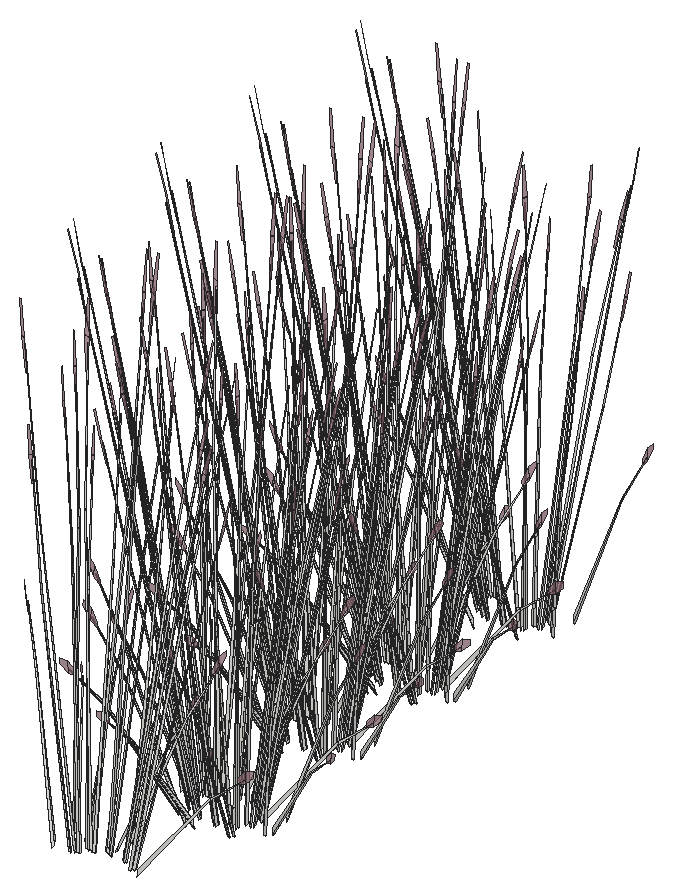
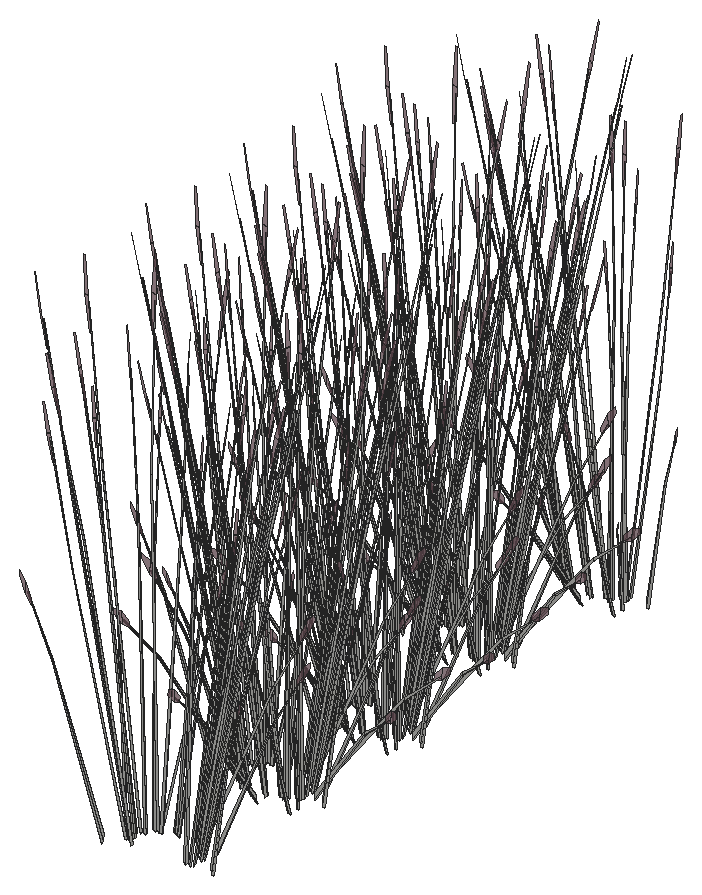
# SketchUp Ruby script. Lengths in inches.
U = 1.inch
M = Sketchup.active_model
def pt(a) = Geom::Point3d.new(a.map { |v| v * U })
def face(e, loops, mat)
  f = e.add_face(loops[0].map { |a| pt(a) })
  loops[1..].each { |l| e.add_face(l.map { |a| pt(a) }).erase! }
  f.material = f.back_material = mat if mat
  f
end
# faces: each face lists its corners as indices into pts; further lists are holes
def faces(e, pts, list, mat = nil) = list.each { |f| face(e, (f[0].is_a?(Array) ? f : [f]).map { |l| l.map { |i| pts[i] } }, mat) }
# xy, xz, yz: faces in a plane at the given z, y or x. An outline is a flat list of corners, or four numbers for a rectangle; further outlines are holes
def ring(l) = l.size == 4 ? [[l[0], l[1]], [l[2], l[1]], [l[2], l[3]], [l[0], l[3]]] : l.each_slice(2).to_a
def flat(e, list, mat, &to3) = list.each { |f| face(e, (f[0].is_a?(Array) ? f : [f]).map { |l| ring(l).map { |u, v| to3.(u, v) } }, mat) }
def xy(e, z, list, mat = nil) = flat(e, list, mat) { |x, y| [x, y, z] }
def xz(e, y, list, mat = nil) = flat(e, list, mat) { |x, z| [x, y, z] }
def yz(e, x, list, mat = nil) = flat(e, list, mat) { |y, z| [x, y, z] }
def lines(e, pts, list) = list.each { |a, b| e.add_line(pt(pts[a]), pt(pts[b])) }
# prism: a flat outline (further loops are holes) pulled along v
def prism(e, loops, v, mat = nil)
  f = face(e, loops, mat); d = Geom::Vector3d.new(v.map { |x| x * U })
  f.pushpull(f.normal.samedirection?(d) ? d.length : -d.length)
end
def box(e, o, s, mat = nil) = prism(e, [[o, [o[0] + s[0], o[1], o[2]], [o[0] + s[0], o[1] + s[1], o[2]], [o[0], o[1] + s[1], o[2]]]], [0, 0, s[2]], mat)
def at(x, y, z, deg = 0) = Geom::Transformation.translation(pt([x, y, z])) * Geom::Transformation.rotation(ORIGIN, Z_AXIS, deg.degrees)
def axes(o, x, y, z) = Geom::Transformation.new([*x, 0, *y, 0, *z, 0, *pt(o).to_a, 1])
def part(name) = M.definitions.add(name)
# library, detail: a bought-in or finely detailed component or shape, given as its bounding box
def library(name, o, s) = part(name).tap { |d| box(d.entities, o, s) }
def detail(e, o, s) = box(e.add_group.entities, o, s)
def put(e, d, t, mat = nil) = e.add_instance(d, t).tap { |i| i.material = mat if mat }
def group(e, t, mat = nil) = e.add_group.tap { |g| g.transformation = t; g.material = mat if mat }.entities
root = M.entities
M.materials.add("LightPink_Translucent").color = [144, 107, 117]
M.materials["LightPink_Translucent"].alpha = 0.75
c1 = part("blade")
p = [[2.15,0.21,22],[0,0.17,0],[0.09,0.45,0],[2.18,0.31,22],[2.29,0.31,22],[0.38,0.45,0],
  [2.48,0.24,33],[2.49,0.24,33],[2.48,0.22,33]]
faces(c1.entities,p,[[0,1,2,3],[4,5,2,3],[6,3,4,7],[8,0,3,6]])
c2 = part("seeds")
p = [[0.3,-0.1,1.38],[-0.01,-0.03,1.59],[-0.01,-0.03,0.03],[0.14,-0.07,-0.07],[0.29,-0.03,3],[0.15,0.01,3.11]]
faces(c2.entities,p,[[0,1,2,3],[1,0,4,5]],"LightPink_Translucent")
c3 = part("blade with seeds")
put(c3.entities,c1,at(0,0,0))
put(c3.entities,c2,axes([2.4,0.25,30.99],[1.5799,-0.05474,1.17369],[-0.12525,1.92788,0.29478],[-0.07173,-0.02425,1.56792]))
put(root,c3,axes([335.36,424.53,52.46],[-0.28729,-0.24465,0.31292],[0.32804,-0.23159,-0.40398],[0.16667,0.03524,0.77298]))
put(root,c3,axes([335.88,424.44,52.17],[0.10831,-0.00661,1.54581],[0.29709,-0.30358,-0.24447],[0.19266,0.04007,0.12397]))
put(root,c3,axes([331.55,424.15,52.18],[-0.12522,-0.35963,0.42415],[0.49122,-0.06241,0.34973],[-0.14477,0.08458,0.87768]))
put(root,c3,axes([331.45,424.08,52.18],[-0.34663,-0.16434,0.05682],[0.20181,-0.23402,0.44729],[-0.11113,0.07566,0.68204]))
put(root,c3,axes([331.85,424.03,52.46],[0.43951,-0.05584,0.31292],[0.11606,0.31924,-0.40398],[-0.12595,0.08575,0.77298]))
put(root,c3,axes([330.16,423.88,52.16],[0.06444,0.01048,1.56736],[0.19934,0.34525,-0.1481],[-0.13191,0.09062,0.27737]))
put(root,c3,axes([335.62,424.75,52.18],[-0.02542,0.29714,0.05682],[-0.38391,-0.00815,0.44729],[0.14706,0.03109,0.68204]))
put(root,c3,axes([335.65,424.65,52.18],[-0.3723,0.25748,0.42415],[-0.32109,-0.27343,0.34973],[0.17467,0.04749,0.87768]))
put(root,c3,axes([330.85,424.93,52.99],[0.44556,0.1043,-0.05733],[-0.13706,0.32103,-0.25992],[-0.07288,0.04874,0.85731]))
put(root,c3,axes([334.47,424.95,52.46],[-0.07798,-0.31474,0.31292],[0.44579,-0.08311,-0.40398],[0.11974,0.09019,0.77298]))
put(root,c3,axes([332.45,424.66,52.46],[0.34164,-0.20573,0.31292],[0.3234,0.23491,-0.40398],[-0.04921,0.11936,0.77298]))
put(root,c3,axes([334.04,425.39,52.16],[0.00149,-0.04731,1.56736],[0.4327,-0.20872,-0.1481],[0.1503,0.0745,0.27737]))
put(root,c3,axes([332.14,424.85,52.18],[-0.41493,-0.01821,0.05682],[0.01138,-0.27493,0.44729],[-0.04342,0.10531,0.68204]))
put(root,c3,axes([332.27,424.875,52.18],[-0.35954,-0.26661,0.42415],[0.38183,-0.22994,0.34973],[-0.06632,0.12508,0.87768]))
put(root,c3,axes([333.4,425,52.46],[0.15222,-0.30049,0.31292],[0.44409,0.08764,-0.40398],[0.04072,0.12098,0.77298]))
put(root,c3,axes([334.54,425.24,52.18],[-0.22948,0.24822,0.05682],[-0.32679,-0.14452,0.44729],[0.10565,0.07958,0.68204]))
put(root,c3,axes([334,426.07,52.99],[0.34892,-0.22417,-0.05733],[0.3197,0.24551,-0.25992],[0.02251,0.06957,0.85731]))
put(root,c3,axes([334.64,425.17,52.18],[-0.5022,0.08967,0.42415],[-0.08716,-0.35177,0.34973],[0.11811,0.10367,0.87768]))
put(root,c3,axes([333.27,425.27,52.18],[-0.37205,0.1328,0.05682],[-0.18211,-0.24217,0.44729],[0.03593,0.10675,0.68204]))
put(root,c3,axes([331.09,424.89,52.17],[-0.01255,0.07733,1.54581],[0.35618,0.269,-0.24447],[-0.09325,0.12721,0.12397]))
put(root,c3,axes([332.23,424.72,52.77],[0.55492,0.01936,-0.11927],[-0.01517,0.36657,-0.66198],[-0.03855,0.14118,1.00587]))
put(root,c3,axes([333.4,425.25,52.47],[-0.49753,-0.10215,0.47081],[0.17013,-0.33585,0.3882],[0.0299,0.13207,0.97422]))
put(root,c3,axes([331.05,425.6875,52.16],[0.05728,-0.02359,1.56736],[0.47345,0.15692,-0.1481],[-0.01113,0.13066,0.27737]))
put(root,c3,axes([335.16,430.65,52.17],[-0.07723,-0.05479,1.54581],[-0.51538,0.03473,-0.24447],[-0.08225,-0.13104,0.12397]))
put(root,c3,axes([333.14,425.85,52.17],[0.064,0.06292,1.54581],[0.51651,0.02472,-0.24447],[0.05194,0.13877,0.12397]))
put(root,c3,axes([337.48,431.32,52.17],[-0.00487,-0.07777,1.54581],[-0.41166,-0.22476,-0.24447],[0.06364,-0.13625,0.12397]))
put(root,c3,axes([337.37,431.04,52.16],[-0.05128,0.02985,1.56736],[-0.5024,-0.1007,-0.1481],[-0.01819,-0.13025,0.27737]))
put(root,c3,axes([334.63,430.47,52.16],[-0.00942,0.04684,1.56736],[-0.46458,0.16998,-0.1481],[-0.13671,-0.08689,0.27737]))
put(root,c3,axes([334.53,431.3,52.5],[0.56246,-0.10044,0.47505],[0.09762,0.39398,0.3917],[-0.13228,-0.11611,0.983]))
put(root,c3,axes([335.8,431.375,52.18],[0.49753,0.10215,0.42415],[-0.17013,0.33585,0.34973],[-0.0299,-0.13207,0.87768]))
put(root,c3,axes([335.93,431.35,52.18],[0.37205,-0.1328,0.05682],[0.18211,0.24217,0.44729],[-0.03593,-0.10675,0.68204]))
put(root,c3,axes([334.66,431.39,52.18],[0.22948,-0.24822,0.05682],[0.32679,0.14452,0.44729],[-0.10565,-0.07958,0.68204]))
put(root,c3,axes([335.8,431.62,52.46],[-0.15222,0.30049,0.31292],[-0.44409,-0.08764,-0.40398],[-0.04072,-0.12098,0.77298]))
put(root,c3,axes([336.93,431.75,52.18],[0.35954,0.26661,0.42415],[-0.38183,0.22994,0.34973],[0.06632,-0.12508,0.87768]))
put(root,c3,axes([334.76,431.36,52.8],[-0.33698,0.3746,-0.12034],[-0.48801,-0.21581,-0.66795],[-0.16964,-0.10584,1.01494]))
put(root,c3,axes([337.0625,431.77,52.18],[0.41493,0.01821,0.05682],[-0.01138,0.27493,0.44729],[0.04342,-0.10531,0.68204]))
put(root,c3,axes([336.75,431.96,52.46],[-0.34164,0.20573,0.31292],[-0.3234,-0.23491,-0.40398],[0.04921,-0.11936,0.77298]))
put(root,c3,axes([333.47,431.25,52.17],[-0.10864,-0.00276,1.54581],[-0.34587,0.27582,-0.24447],[-0.18454,-0.05636,0.12397]))
put(root,c3,axes([334.73,431.67,52.46],[0.07798,0.31474,0.31292],[-0.44579,0.08311,-0.40398],[-0.11974,-0.09019,0.77298]))
put(root,c3,axes([333.39,431.875,52.5],[0.41698,-0.28837,0.47505],[0.35962,0.30624,0.3917],[-0.19563,-0.05319,0.983]))
put(root,c3,axes([338.73,432.53,52.16],[-0.06595,-0.00297,1.56736],[-0.27386,-0.31799,-0.1481],[0.10998,-0.10455,0.27737]))
put(root,c3,axes([333.58,431.875,52.18],[0.02542,-0.29714,0.05682],[0.38391,0.00815,0.44729],[-0.14706,-0.03109,0.68204]))
put(root,c3,axes([337.35,432.6,52.46],[-0.43951,0.05584,0.31292],[-0.11606,-0.31924,-0.40398],[0.12595,-0.08575,0.77298]))
put(root,c3,axes([337.75,432.54,52.18],[0.34663,0.16434,0.05682],[-0.20181,0.23402,0.44729],[0.11113,-0.07566,0.68204]))
put(root,c3,axes([337.65,432.48,52.18],[0.12522,0.35963,0.42415],[-0.49122,0.06241,0.34973],[0.14477,-0.08458,0.87768]))
put(root,c3,axes([338.97,432.91,52.17],[0.07006,-0.05952,1.54581],[-0.08968,-0.3651,-0.24447],[0.1758,-0.06922,0.12397]))
put(root,c3,axes([333.05,431.49,52.16],[0.03743,0.039,1.56736],[-0.18045,0.35054,-0.1481],[-0.18276,0.00254,0.27737]))
put(root,c3,axes([333.84,432.1,52.46],[0.28729,0.24465,0.31292],[-0.32804,0.23159,-0.40398],[-0.16667,-0.03524,0.77298]))
put(root,c3,axes([337.42,433.36,52.46],[-0.41962,-0.10901,0.31292],[0.12239,-0.31802,-0.40398],[0.16894,-0.02916,0.77298]))
put(root,c3,axes([333.02,432.78,52.18],[0.14265,-0.35629,0.42415],[0.46898,0.12183,0.34973],[-0.18443,0.02141,0.87768]))
put(root,c3,axes([332.99,432.68,52.18],[-0.18545,-0.26643,0.05682],[0.33817,-0.13041,0.44729],[-0.14907,0.02573,0.68204]))
put(root,c3,axes([337.8,433.46,52.18],[0.18545,0.26643,0.05682],[-0.33817,0.13041,0.44729],[0.14907,-0.02573,0.68204]))
put(root,c3,axes([337.76,433.36,52.18],[-0.14265,0.35629,0.42415],[-0.46898,-0.12183,0.34973],[0.18443,-0.02141,0.87768]))
put(root,c3,axes([333.37,432.78,52.46],[0.41962,0.10901,0.31292],[-0.12239,0.31802,-0.40398],[-0.16894,0.02916,0.77298]))
put(root,c3,axes([338.6,434.52,52.16],[-0.04566,-0.03421,1.56736],[0.09987,-0.36669,-0.1481],[0.17984,-0.02343,0.27737]))
put(root,c3,axes([332.66,433.03,52.17],[-0.08245,0.05073,1.54581],[0.00701,0.37067,-0.24447],[-0.18899,0.0482,0.12397]))
put(root,c3,axes([336.95,434.04,52.46],[-0.28729,-0.24465,0.31292],[0.32804,-0.23159,-0.40398],[0.16667,0.03524,0.77298]))
put(root,c3,axes([337.47,433.96,52.17],[0.10831,-0.00661,1.54581],[0.29709,-0.30358,-0.24447],[0.19266,0.04007,0.12397]))
put(root,c3,axes([333.14,433.66,52.18],[-0.12522,-0.35963,0.42415],[0.49122,-0.06241,0.34973],[-0.14477,0.08458,0.87768]))
put(root,c3,axes([333.04,433.6,52.18],[-0.34663,-0.16434,0.05682],[0.20181,-0.23402,0.44729],[-0.11113,0.07566,0.68204]))
put(root,c3,axes([333.4375,433.55,52.46],[0.43951,-0.05584,0.31292],[0.11606,0.31924,-0.40398],[-0.12595,0.08575,0.77298]))
put(root,c3,axes([331.75,433.4,52.16],[0.06444,0.01048,1.56736],[0.19934,0.34525,-0.1481],[-0.13191,0.09062,0.27737]))
put(root,c3,axes([337.21,434.27,52.18],[-0.02542,0.29714,0.05682],[-0.38391,-0.00815,0.44729],[0.14706,0.03109,0.68204]))
put(root,c3,axes([337.24,434.17,52.18],[-0.3723,0.25748,0.42415],[-0.32109,-0.27343,0.34973],[0.17467,0.04749,0.87768]))
put(root,c3,axes([332.44,434.45,52.99],[0.44556,0.1043,-0.05733],[-0.13706,0.32103,-0.25992],[-0.07288,0.04874,0.85731]))
put(root,c3,axes([336.06,434.47,52.46],[-0.07798,-0.31474,0.31292],[0.44579,-0.08311,-0.40398],[0.11974,0.09019,0.77298]))
put(root,c3,axes([334.03,434.18,52.46],[0.34164,-0.20573,0.31292],[0.3234,0.23491,-0.40398],[-0.04921,0.11936,0.77298]))
put(root,c3,axes([335.62,434.91,52.16],[0.00149,-0.04731,1.56736],[0.4327,-0.20872,-0.1481],[0.1503,0.0745,0.27737]))
put(root,c3,axes([333.72,434.37,52.18],[-0.41493,-0.01821,0.05682],[0.01138,-0.27493,0.44729],[-0.04342,0.10531,0.68204]))
put(root,c3,axes([333.86,434.39,52.18],[-0.35954,-0.26661,0.42415],[0.38183,-0.22994,0.34973],[-0.06632,0.12508,0.87768]))
put(root,c3,axes([334.99,434.52,52.46],[0.15222,-0.30049,0.31292],[0.44409,0.08764,-0.40398],[0.04072,0.12098,0.77298]))
put(root,c3,axes([336.13,434.75,52.18],[-0.22948,0.24822,0.05682],[-0.32679,-0.14452,0.44729],[0.10565,0.07958,0.68204]))
put(root,c3,axes([335.59,435.59,52.99],[0.34892,-0.22417,-0.05733],[0.3197,0.24551,-0.25992],[0.02251,0.06957,0.85731]))
put(root,c3,axes([336.22,434.6875,52.18],[-0.5022,0.08967,0.42415],[-0.08716,-0.35177,0.34973],[0.11811,0.10367,0.87768]))
put(root,c3,axes([334.85,434.79,52.18],[-0.37205,0.1328,0.05682],[-0.18211,-0.24217,0.44729],[0.03593,0.10675,0.68204]))
put(root,c3,axes([332.68,434.41,52.17],[-0.01255,0.07733,1.54581],[0.35618,0.269,-0.24447],[-0.09325,0.12721,0.12397]))
put(root,c3,axes([333.82,434.24,52.77],[0.55492,0.01936,-0.11927],[-0.01517,0.36657,-0.66198],[-0.03855,0.14118,1.00587]))
put(root,c3,axes([334.98,434.77,52.47],[-0.49753,-0.10215,0.47081],[0.17013,-0.33585,0.3882],[0.0299,0.13207,0.97422]))
put(root,c3,axes([332.64,435.2,52.16],[0.05728,-0.02359,1.56736],[0.47345,0.15692,-0.1481],[-0.01113,0.13066,0.27737]))
put(root,c3,axes([334.73,435.37,52.17],[0.064,0.06292,1.54581],[0.51651,0.02472,-0.24447],[0.05194,0.13877,0.12397]))
put(root,c3,axes([333.57,440.52,52.17],[-0.07723,-0.05479,1.54581],[-0.51538,0.03473,-0.24447],[-0.08225,-0.13104,0.12397]))
put(root,c3,axes([335.89,441.1875,52.17],[-0.00487,-0.07777,1.54581],[-0.41166,-0.22476,-0.24447],[0.06364,-0.13625,0.12397]))
put(root,c3,axes([335.78,440.91,52.16],[-0.05128,0.02985,1.56736],[-0.5024,-0.1007,-0.1481],[-0.01819,-0.13025,0.27737]))
put(root,c3,axes([333.05,440.34,52.16],[-0.00942,0.04684,1.56736],[-0.46458,0.16998,-0.1481],[-0.13671,-0.08689,0.27737]))
put(root,c3,axes([332.94,441.17,52.5],[0.56246,-0.10044,0.47505],[0.09762,0.39398,0.3917],[-0.13228,-0.11611,0.983]))
put(root,c3,axes([334.22,441.24,52.18],[0.49753,0.10215,0.42415],[-0.17013,0.33585,0.34973],[-0.0299,-0.13207,0.87768]))
put(root,c3,axes([334.35,441.22,52.18],[0.37205,-0.1328,0.05682],[0.18211,0.24217,0.44729],[-0.03593,-0.10675,0.68204]))
put(root,c3,axes([333.07,441.25,52.18],[0.22948,-0.24822,0.05682],[0.32679,0.14452,0.44729],[-0.10565,-0.07958,0.68204]))
put(root,c3,axes([334.21,441.49,52.46],[-0.15222,0.30049,0.31292],[-0.44409,-0.08764,-0.40398],[-0.04072,-0.12098,0.77298]))
put(root,c3,axes([335.34,441.61,52.18],[0.35954,0.26661,0.42415],[-0.38183,0.22994,0.34973],[0.06632,-0.12508,0.87768]))
put(root,c3,axes([333.18,441.23,52.8],[-0.33698,0.3746,-0.12034],[-0.48801,-0.21581,-0.66795],[-0.16964,-0.10584,1.01494]))
put(root,c3,axes([335.48,441.64,52.18],[0.41493,0.01821,0.05682],[-0.01138,0.27493,0.44729],[0.04342,-0.10531,0.68204]))
put(root,c3,axes([335.17,441.83,52.46],[-0.34164,0.20573,0.31292],[-0.3234,-0.23491,-0.40398],[0.04921,-0.11936,0.77298]))
put(root,c3,axes([331.88,441.12,52.17],[-0.10864,-0.00276,1.54581],[-0.34587,0.27582,-0.24447],[-0.18454,-0.05636,0.12397]))
put(root,c3,axes([333.14,441.54,52.46],[0.07798,0.31474,0.31292],[-0.44579,0.08311,-0.40398],[-0.11974,-0.09019,0.77298]))
put(root,c3,axes([331.8,441.74,52.5],[0.41698,-0.28837,0.47505],[0.35962,0.30624,0.3917],[-0.19563,-0.05319,0.983]))
put(root,c3,axes([337.14,442.4,52.16],[-0.06595,-0.00297,1.56736],[-0.27386,-0.31799,-0.1481],[0.10998,-0.10455,0.27737]))
put(root,c3,axes([331.99,441.74,52.18],[0.02542,-0.29714,0.05682],[0.38391,0.00815,0.44729],[-0.14706,-0.03109,0.68204]))
put(root,c3,axes([335.76,442.46,52.46],[-0.43951,0.05584,0.31292],[-0.11606,-0.31924,-0.40398],[0.12595,-0.08575,0.77298]))
put(root,c3,axes([336.16,442.41,52.18],[0.34663,0.16434,0.05682],[-0.20181,0.23402,0.44729],[0.11113,-0.07566,0.68204]))
put(root,c3,axes([336.0625,442.34,52.18],[0.12522,0.35963,0.42415],[-0.49122,0.06241,0.34973],[0.14477,-0.08458,0.87768]))
put(root,c3,axes([337.39,442.78,52.17],[0.07006,-0.05952,1.54581],[-0.08968,-0.3651,-0.24447],[0.1758,-0.06922,0.12397]))
put(root,c3,axes([331.47,441.35,52.16],[0.03743,0.039,1.56736],[-0.18045,0.35054,-0.1481],[-0.18276,0.00254,0.27737]))
put(root,c3,axes([332.25,441.96,52.46],[0.28729,0.24465,0.31292],[-0.32804,0.23159,-0.40398],[-0.16667,-0.03524,0.77298]))
put(root,c3,axes([335.83,443.23,52.46],[-0.41962,-0.10901,0.31292],[0.12239,-0.31802,-0.40398],[0.16894,-0.02916,0.77298]))
put(root,c3,axes([331.4375,442.64,52.18],[0.14265,-0.35629,0.42415],[0.46898,0.12183,0.34973],[-0.18443,0.02141,0.87768]))
put(root,c3,axes([331.4,442.55,52.18],[-0.18545,-0.26643,0.05682],[0.33817,-0.13041,0.44729],[-0.14907,0.02573,0.68204]))
put(root,c3,axes([336.21,443.32,52.18],[0.18545,0.26643,0.05682],[-0.33817,0.13041,0.44729],[0.14907,-0.02573,0.68204]))
put(root,c3,axes([336.18,443.23,52.18],[-0.14265,0.35629,0.42415],[-0.46898,-0.12183,0.34973],[0.18443,-0.02141,0.87768]))
put(root,c3,axes([331.78,442.65,52.46],[0.41962,0.10901,0.31292],[-0.12239,0.31802,-0.40398],[-0.16894,0.02916,0.77298]))
put(root,c3,axes([337.02,444.38,52.16],[-0.04566,-0.03421,1.56736],[0.09987,-0.36669,-0.1481],[0.17984,-0.02343,0.27737]))
put(root,c3,axes([331.08,442.9,52.17],[-0.08245,0.05073,1.54581],[0.00701,0.37067,-0.24447],[-0.18899,0.0482,0.12397]))
put(root,c3,axes([335.36,443.91,52.46],[-0.28729,-0.24465,0.31292],[0.32804,-0.23159,-0.40398],[0.16667,0.03524,0.77298]))
put(root,c3,axes([335.88,443.83,52.17],[0.10831,-0.00661,1.54581],[0.29709,-0.30358,-0.24447],[0.19266,0.04007,0.12397]))
put(root,c3,axes([331.55,443.53,52.18],[-0.12522,-0.35963,0.42415],[0.49122,-0.06241,0.34973],[-0.14477,0.08458,0.87768]))
put(root,c3,axes([331.45,443.46,52.18],[-0.34663,-0.16434,0.05682],[0.20181,-0.23402,0.44729],[-0.11113,0.07566,0.68204]))
put(root,c3,axes([331.85,443.41,52.46],[0.43951,-0.05584,0.31292],[0.11606,0.31924,-0.40398],[-0.12595,0.08575,0.77298]))
put(root,c3,axes([330.16,443.27,52.16],[0.06444,0.01048,1.56736],[0.19934,0.34525,-0.1481],[-0.13191,0.09062,0.27737]))
put(root,c3,axes([335.62,444.13,52.18],[-0.02542,0.29714,0.05682],[-0.38391,-0.00815,0.44729],[0.14706,0.03109,0.68204]))
put(root,c3,axes([335.65,444.04,52.18],[-0.3723,0.25748,0.42415],[-0.32109,-0.27343,0.34973],[0.17467,0.04749,0.87768]))
put(root,c3,axes([330.85,444.32,52.99],[0.44556,0.1043,-0.05733],[-0.13706,0.32103,-0.25992],[-0.07288,0.04874,0.85731]))
put(root,c3,axes([334.47,444.34,52.46],[-0.07798,-0.31474,0.31292],[0.44579,-0.08311,-0.40398],[0.11974,0.09019,0.77298]))
put(root,c3,axes([332.45,444.05,52.46],[0.34164,-0.20573,0.31292],[0.3234,0.23491,-0.40398],[-0.04921,0.11936,0.77298]))
put(root,c3,axes([334.04,444.78,52.16],[0.00149,-0.04731,1.56736],[0.4327,-0.20872,-0.1481],[0.1503,0.0745,0.27737]))
put(root,c3,axes([332.14,444.23,52.18],[-0.41493,-0.01821,0.05682],[0.01138,-0.27493,0.44729],[-0.04342,0.10531,0.68204]))
put(root,c3,axes([332.27,444.26,52.18],[-0.35954,-0.26661,0.42415],[0.38183,-0.22994,0.34973],[-0.06632,0.12508,0.87768]))
put(root,c3,axes([333.4,444.39,52.46],[0.15222,-0.30049,0.31292],[0.44409,0.08764,-0.40398],[0.04072,0.12098,0.77298]))
put(root,c3,axes([334.54,444.62,52.18],[-0.22948,0.24822,0.05682],[-0.32679,-0.14452,0.44729],[0.10565,0.07958,0.68204]))
put(root,c3,axes([333.57,448.89,52.17],[-0.07723,-0.05479,1.54581],[-0.51538,0.03473,-0.24447],[-0.08225,-0.13104,0.12397]))
put(root,c3,axes([334,445.46,52.99],[0.34892,-0.22417,-0.05733],[0.3197,0.24551,-0.25992],[0.02251,0.06957,0.85731]))
put(root,c3,axes([334.64,444.55,52.18],[-0.5022,0.08967,0.42415],[-0.08716,-0.35177,0.34973],[0.11811,0.10367,0.87768]))
put(root,c3,axes([333.27,444.66,52.18],[-0.37205,0.1328,0.05682],[-0.18211,-0.24217,0.44729],[0.03593,0.10675,0.68204]))
put(root,c3,axes([331.09,444.28,52.17],[-0.01255,0.07733,1.54581],[0.35618,0.269,-0.24447],[-0.09325,0.12721,0.12397]))
put(root,c3,axes([332.23,444.1,52.77],[0.55492,0.01936,-0.11927],[-0.01517,0.36657,-0.66198],[-0.03855,0.14118,1.00587]))
put(root,c3,axes([333.4,444.63,52.47],[-0.49753,-0.10215,0.47081],[0.17013,-0.33585,0.3882],[0.0299,0.13207,0.97422]))
put(root,c3,axes([335.89,449.56,52.17],[-0.00487,-0.07777,1.54581],[-0.41166,-0.22476,-0.24447],[0.06364,-0.13625,0.12397]))
put(root,c3,axes([335.78,449.28,52.16],[-0.05128,0.02985,1.56736],[-0.5024,-0.1007,-0.1481],[-0.01819,-0.13025,0.27737]))
put(root,c3,axes([333.05,448.71,52.16],[-0.00942,0.04684,1.56736],[-0.46458,0.16998,-0.1481],[-0.13671,-0.08689,0.27737]))
put(root,c3,axes([332.94,449.54,52.5],[0.56246,-0.10044,0.47505],[0.09762,0.39398,0.3917],[-0.13228,-0.11611,0.983]))
put(root,c3,axes([331.05,445.07,52.16],[0.05728,-0.02359,1.56736],[0.47345,0.15692,-0.1481],[-0.01113,0.13066,0.27737]))
put(root,c3,axes([334.22,449.61,52.18],[0.49753,0.10215,0.42415],[-0.17013,0.33585,0.34973],[-0.0299,-0.13207,0.87768]))
put(root,c3,axes([334.35,449.59,52.18],[0.37205,-0.1328,0.05682],[0.18211,0.24217,0.44729],[-0.03593,-0.10675,0.68204]))
put(root,c3,axes([333.14,445.24,52.17],[0.064,0.06292,1.54581],[0.51651,0.02472,-0.24447],[0.05194,0.13877,0.12397]))
put(root,c3,axes([333.07,449.625,52.18],[0.22948,-0.24822,0.05682],[0.32679,0.14452,0.44729],[-0.10565,-0.07958,0.68204]))
put(root,c3,axes([334.21,449.86,52.46],[-0.15222,0.30049,0.31292],[-0.44409,-0.08764,-0.40398],[-0.04072,-0.12098,0.77298]))
put(root,c3,axes([335.34,449.99,52.18],[0.35954,0.26661,0.42415],[-0.38183,0.22994,0.34973],[0.06632,-0.12508,0.87768]))
put(root,c3,axes([333.18,449.6,52.8],[-0.33698,0.3746,-0.12034],[-0.48801,-0.21581,-0.66795],[-0.16964,-0.10584,1.01494]))
put(root,c3,axes([335.48,450.01,52.18],[0.41493,0.01821,0.05682],[-0.01138,0.27493,0.44729],[0.04342,-0.10531,0.68204]))
put(root,c3,axes([335.17,450.2,52.46],[-0.34164,0.20573,0.31292],[-0.3234,-0.23491,-0.40398],[0.04921,-0.11936,0.77298]))
put(root,c3,axes([331.88,449.49,52.17],[-0.10864,-0.00276,1.54581],[-0.34587,0.27582,-0.24447],[-0.18454,-0.05636,0.12397]))
put(root,c3,axes([333.14,449.91,52.46],[0.07798,0.31474,0.31292],[-0.44579,0.08311,-0.40398],[-0.11974,-0.09019,0.77298]))
put(root,c3,axes([331.8,450.12,52.5],[0.41698,-0.28837,0.47505],[0.35962,0.30624,0.3917],[-0.19563,-0.05319,0.983]))
put(root,c3,axes([337.14,450.77,52.16],[-0.06595,-0.00297,1.56736],[-0.27386,-0.31799,-0.1481],[0.10998,-0.10455,0.27737]))
put(root,c3,axes([331.99,450.11,52.18],[0.02542,-0.29714,0.05682],[0.38391,0.00815,0.44729],[-0.14706,-0.03109,0.68204]))
put(root,c3,axes([335.76,450.83,52.46],[-0.43951,0.05584,0.31292],[-0.11606,-0.31924,-0.40398],[0.12595,-0.08575,0.77298]))
put(root,c3,axes([336.16,450.78,52.18],[0.34663,0.16434,0.05682],[-0.20181,0.23402,0.44729],[0.11113,-0.07566,0.68204]))
put(root,c3,axes([336.0625,450.72,52.18],[0.12522,0.35963,0.42415],[-0.49122,0.06241,0.34973],[0.14477,-0.08458,0.87768]))
put(root,c3,axes([337.39,451.15,52.17],[0.07006,-0.05952,1.54581],[-0.08968,-0.3651,-0.24447],[0.1758,-0.06922,0.12397]))
put(root,c3,axes([331.47,449.73,52.16],[0.03743,0.039,1.56736],[-0.18045,0.35054,-0.1481],[-0.18276,0.00254,0.27737]))
put(root,c3,axes([332.25,450.34,52.46],[0.28729,0.24465,0.31292],[-0.32804,0.23159,-0.40398],[-0.16667,-0.03524,0.77298]))
put(root,c3,axes([335.83,451.6,52.46],[-0.41962,-0.10901,0.31292],[0.12239,-0.31802,-0.40398],[0.16894,-0.02916,0.77298]))
put(root,c3,axes([331.4375,451.02,52.18],[0.14265,-0.35629,0.42415],[0.46898,0.12183,0.34973],[-0.18443,0.02141,0.87768]))
put(root,c3,axes([331.4,450.92,52.18],[-0.18545,-0.26643,0.05682],[0.33817,-0.13041,0.44729],[-0.14907,0.02573,0.68204]))
put(root,c3,axes([336.21,451.7,52.18],[0.18545,0.26643,0.05682],[-0.33817,0.13041,0.44729],[0.14907,-0.02573,0.68204]))
put(root,c3,axes([336.18,451.6,52.18],[-0.14265,0.35629,0.42415],[-0.46898,-0.12183,0.34973],[0.18443,-0.02141,0.87768]))
put(root,c3,axes([331.78,451.02,52.46],[0.41962,0.10901,0.31292],[-0.12239,0.31802,-0.40398],[-0.16894,0.02916,0.77298]))
put(root,c3,axes([337.02,452.76,52.16],[-0.04566,-0.03421,1.56736],[0.09987,-0.36669,-0.1481],[0.17984,-0.02343,0.27737]))
put(root,c3,axes([331.08,451.27,52.17],[-0.08245,0.05073,1.54581],[0.00701,0.37067,-0.24447],[-0.18899,0.0482,0.12397]))
put(root,c3,axes([335.36,452.28,52.46],[-0.28729,-0.24465,0.31292],[0.32804,-0.23159,-0.40398],[0.16667,0.03524,0.77298]))
put(root,c3,axes([335.88,452.2,52.17],[0.10831,-0.00661,1.54581],[0.29709,-0.30358,-0.24447],[0.19266,0.04007,0.12397]))
put(root,c3,axes([331.55,451.9,52.18],[-0.12522,-0.35963,0.42415],[0.49122,-0.06241,0.34973],[-0.14477,0.08458,0.87768]))
put(root,c3,axes([331.45,451.84,52.18],[-0.34663,-0.16434,0.05682],[0.20181,-0.23402,0.44729],[-0.11113,0.07566,0.68204]))
put(root,c3,axes([331.85,451.78,52.46],[0.43951,-0.05584,0.31292],[0.11606,0.31924,-0.40398],[-0.12595,0.08575,0.77298]))
put(root,c3,axes([330.16,451.64,52.16],[0.06444,0.01048,1.56736],[0.19934,0.34525,-0.1481],[-0.13191,0.09062,0.27737]))
put(root,c3,axes([335.62,452.51,52.18],[-0.02542,0.29714,0.05682],[-0.38391,-0.00815,0.44729],[0.14706,0.03109,0.68204]))
put(root,c3,axes([335.65,452.41,52.18],[-0.3723,0.25748,0.42415],[-0.32109,-0.27343,0.34973],[0.17467,0.04749,0.87768]))
put(root,c3,axes([330.85,452.69,52.99],[0.44556,0.1043,-0.05733],[-0.13706,0.32103,-0.25992],[-0.07288,0.04874,0.85731]))
put(root,c3,axes([334.47,452.71,52.46],[-0.07798,-0.31474,0.31292],[0.44579,-0.08311,-0.40398],[0.11974,0.09019,0.77298]))
put(root,c3,axes([332.45,452.42,52.46],[0.34164,-0.20573,0.31292],[0.3234,0.23491,-0.40398],[-0.04921,0.11936,0.77298]))
put(root,c3,axes([334.04,453.15,52.16],[0.00149,-0.04731,1.56736],[0.4327,-0.20872,-0.1481],[0.1503,0.0745,0.27737]))
put(root,c3,axes([332.14,452.61,52.18],[-0.41493,-0.01821,0.05682],[0.01138,-0.27493,0.44729],[-0.04342,0.10531,0.68204]))
put(root,c3,axes([332.27,452.63,52.18],[-0.35954,-0.26661,0.42415],[0.38183,-0.22994,0.34973],[-0.06632,0.12508,0.87768]))
put(root,c3,axes([333.4,452.76,52.46],[0.15222,-0.30049,0.31292],[0.44409,0.08764,-0.40398],[0.04072,0.12098,0.77298]))
put(root,c3,axes([334.54,452.99,52.18],[-0.22948,0.24822,0.05682],[-0.32679,-0.14452,0.44729],[0.10565,0.07958,0.68204]))
put(root,c3,axes([334,453.83,52.99],[0.34892,-0.22417,-0.05733],[0.3197,0.24551,-0.25992],[0.02251,0.06957,0.85731]))
put(root,c3,axes([334.64,452.93,52.18],[-0.5022,0.08967,0.42415],[-0.08716,-0.35177,0.34973],[0.11811,0.10367,0.87768]))
put(root,c3,axes([333.27,453.03,52.18],[-0.37205,0.1328,0.05682],[-0.18211,-0.24217,0.44729],[0.03593,0.10675,0.68204]))
put(root,c3,axes([331.09,452.65,52.17],[-0.01255,0.07733,1.54581],[0.35618,0.269,-0.24447],[-0.09325,0.12721,0.12397]))
put(root,c3,axes([332.23,452.48,52.77],[0.55492,0.01936,-0.11927],[-0.01517,0.36657,-0.66198],[-0.03855,0.14118,1.00587]))
put(root,c3,axes([333.4,453.01,52.47],[-0.49753,-0.10215,0.47081],[0.17013,-0.33585,0.3882],[0.0299,0.13207,0.97422]))
put(root,c3,axes([331.05,453.44,52.16],[0.05728,-0.02359,1.56736],[0.47345,0.15692,-0.1481],[-0.01113,0.13066,0.27737]))
put(root,c3,axes([333.14,453.61,52.17],[0.064,0.06292,1.54581],[0.51651,0.02472,-0.24447],[0.05194,0.13877,0.12397]))
put(root,c3,axes([335.78,458.8,52.16],[-0.05128,0.02985,1.56736],[-0.5024,-0.1007,-0.1481],[-0.01819,-0.13025,0.27737]))
put(root,c3,axes([333.05,458.22,52.16],[-0.00942,0.04684,1.56736],[-0.46458,0.16998,-0.1481],[-0.13671,-0.08689,0.27737]))
put(root,c3,axes([332.94,459.05,52.5],[0.56246,-0.10044,0.47505],[0.09762,0.39398,0.3917],[-0.13228,-0.11611,0.983]))
put(root,c3,axes([334.22,459.13,52.18],[0.49753,0.10215,0.42415],[-0.17013,0.33585,0.34973],[-0.0299,-0.13207,0.87768]))
put(root,c3,axes([334.35,459.1,52.18],[0.37205,-0.1328,0.05682],[0.18211,0.24217,0.44729],[-0.03593,-0.10675,0.68204]))
put(root,c3,axes([333.07,459.14,52.18],[0.22948,-0.24822,0.05682],[0.32679,0.14452,0.44729],[-0.10565,-0.07958,0.68204]))
put(root,c3,axes([334.21,459.375,52.46],[-0.15222,0.30049,0.31292],[-0.44409,-0.08764,-0.40398],[-0.04072,-0.12098,0.77298]))
put(root,c3,axes([335.34,459.5,52.18],[0.35954,0.26661,0.42415],[-0.38183,0.22994,0.34973],[0.06632,-0.12508,0.87768]))
put(root,c3,axes([333.18,459.11,52.8],[-0.33698,0.3746,-0.12034],[-0.48801,-0.21581,-0.66795],[-0.16964,-0.10584,1.01494]))
put(root,c3,axes([335.48,459.53,52.18],[0.41493,0.01821,0.05682],[-0.01138,0.27493,0.44729],[0.04342,-0.10531,0.68204]))
put(root,c3,axes([335.17,459.71,52.46],[-0.34164,0.20573,0.31292],[-0.3234,-0.23491,-0.40398],[0.04921,-0.11936,0.77298]))
put(root,c3,axes([333.14,459.42,52.46],[0.07798,0.31474,0.31292],[-0.44579,0.08311,-0.40398],[-0.11974,-0.09019,0.77298]))
put(root,c3,axes([331.8,459.63,52.5],[0.41698,-0.28837,0.47505],[0.35962,0.30624,0.3917],[-0.19563,-0.05319,0.983]))
put(root,c3,axes([337.14,460.28,52.16],[-0.06595,-0.00297,1.56736],[-0.27386,-0.31799,-0.1481],[0.10998,-0.10455,0.27737]))
put(root,c3,axes([331.99,459.63,52.18],[0.02542,-0.29714,0.05682],[0.38391,0.00815,0.44729],[-0.14706,-0.03109,0.68204]))
put(root,c3,axes([335.76,460.35,52.46],[-0.43951,0.05584,0.31292],[-0.11606,-0.31924,-0.40398],[0.12595,-0.08575,0.77298]))
put(root,c3,axes([336.16,460.3,52.18],[0.34663,0.16434,0.05682],[-0.20181,0.23402,0.44729],[0.11113,-0.07566,0.68204]))
put(root,c3,axes([336.0625,460.23,52.18],[0.12522,0.35963,0.42415],[-0.49122,0.06241,0.34973],[0.14477,-0.08458,0.87768]))
put(root,c3,axes([331.47,459.24,52.16],[0.03743,0.039,1.56736],[-0.18045,0.35054,-0.1481],[-0.18276,0.00254,0.27737]))
put(root,c3,axes([332.25,459.85,52.46],[0.28729,0.24465,0.31292],[-0.32804,0.23159,-0.40398],[-0.16667,-0.03524,0.77298]))
put(root,c3,axes([335.83,461.11,52.46],[-0.41962,-0.10901,0.31292],[0.12239,-0.31802,-0.40398],[0.16894,-0.02916,0.77298]))
put(root,c3,axes([331.4375,460.53,52.18],[0.14265,-0.35629,0.42415],[0.46898,0.12183,0.34973],[-0.18443,0.02141,0.87768]))
put(root,c3,axes([331.4,460.4375,52.18],[-0.18545,-0.26643,0.05682],[0.33817,-0.13041,0.44729],[-0.14907,0.02573,0.68204]))
put(root,c3,axes([336.21,461.21,52.18],[0.18545,0.26643,0.05682],[-0.33817,0.13041,0.44729],[0.14907,-0.02573,0.68204]))
put(root,c3,axes([336.18,461.12,52.18],[-0.14265,0.35629,0.42415],[-0.46898,-0.12183,0.34973],[0.18443,-0.02141,0.87768]))
put(root,c3,axes([331.78,460.54,52.46],[0.41962,0.10901,0.31292],[-0.12239,0.31802,-0.40398],[-0.16894,0.02916,0.77298]))
put(root,c3,axes([337.02,462.27,52.16],[-0.04566,-0.03421,1.56736],[0.09987,-0.36669,-0.1481],[0.17984,-0.02343,0.27737]))
put(root,c3,axes([335.36,461.8,52.46],[-0.28729,-0.24465,0.31292],[0.32804,-0.23159,-0.40398],[0.16667,0.03524,0.77298]))
put(root,c3,axes([331.55,461.42,52.18],[-0.12522,-0.35963,0.42415],[0.49122,-0.06241,0.34973],[-0.14477,0.08458,0.87768]))
put(root,c3,axes([331.45,461.35,52.18],[-0.34663,-0.16434,0.05682],[0.20181,-0.23402,0.44729],[-0.11113,0.07566,0.68204]))
put(root,c3,axes([331.85,461.3,52.46],[0.43951,-0.05584,0.31292],[0.11606,0.31924,-0.40398],[-0.12595,0.08575,0.77298]))
put(root,c3,axes([330.16,461.16,52.16],[0.06444,0.01048,1.56736],[0.19934,0.34525,-0.1481],[-0.13191,0.09062,0.27737]))
